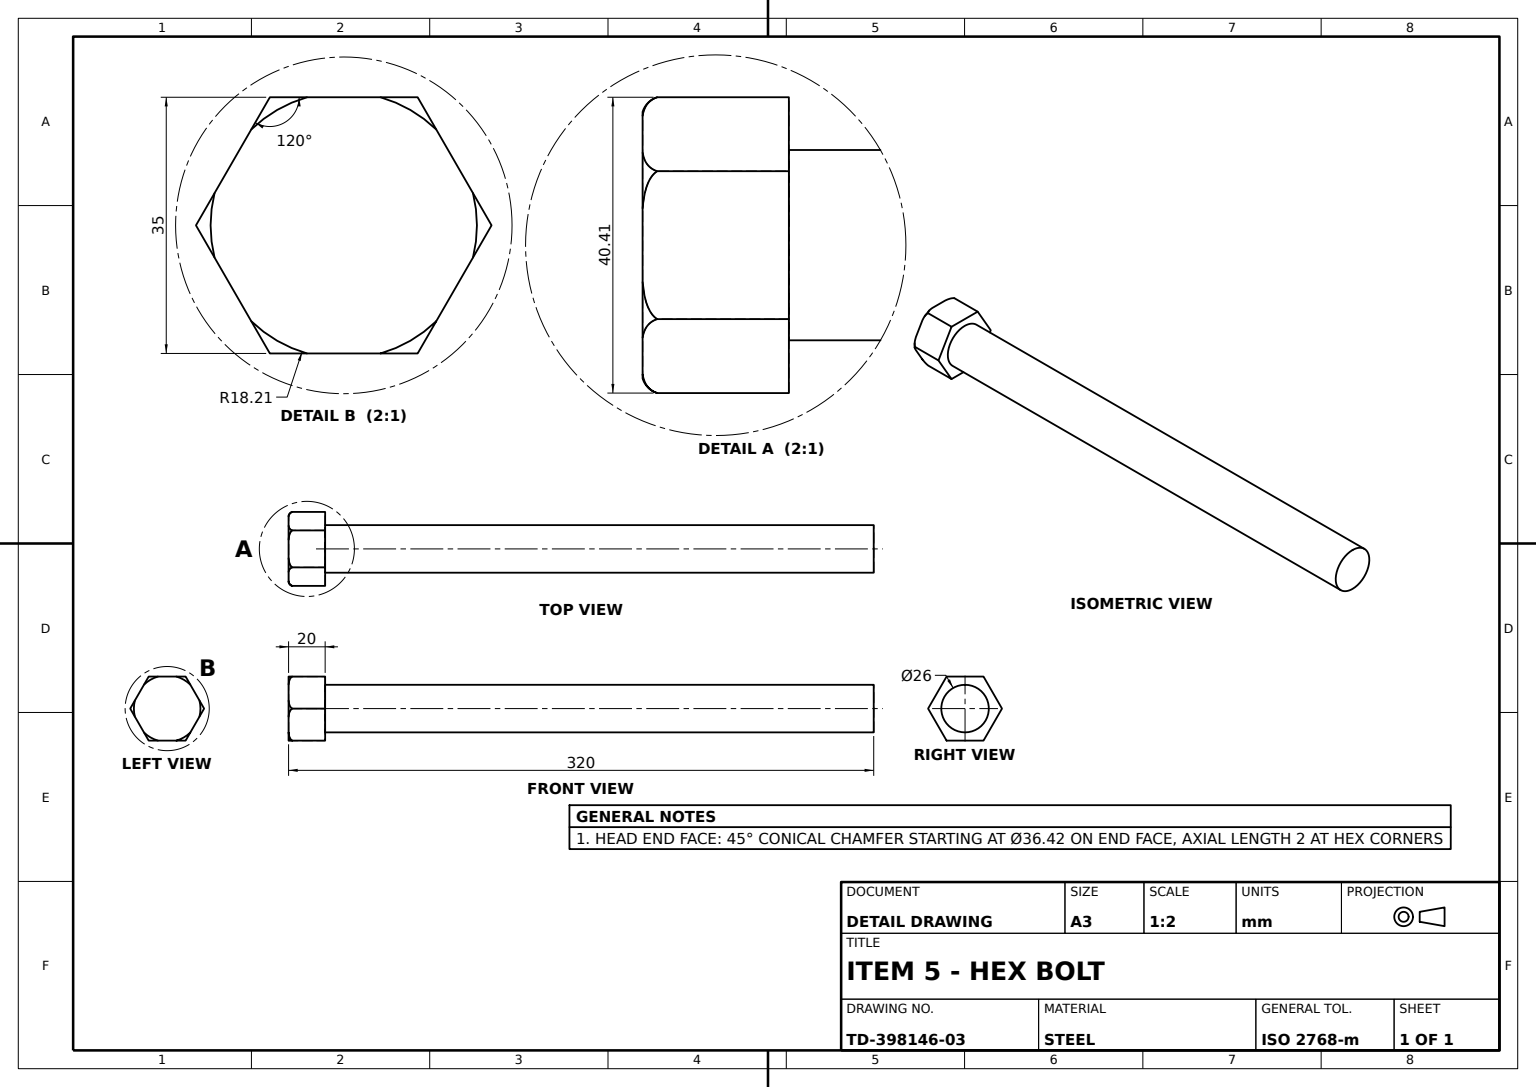
ISO-10303-21;
HEADER;
FILE_DESCRIPTION((''),'2;1');
FILE_NAME('','',(''),(''),'','','');
FILE_SCHEMA(('AUTOMOTIVE_DESIGN'));
ENDSEC;
DATA;
#1=APPLICATION_CONTEXT('');
#2=PRODUCT_CONTEXT('',#1,'mechanical');
#3=PRODUCT('','','',(#2));
#4=PRODUCT_DEFINITION_FORMATION('','',#3);
#5=PRODUCT_DEFINITION_CONTEXT('',#1,'design');
#6=PRODUCT_DEFINITION('','',#4,#5);
#7=PRODUCT_DEFINITION_SHAPE('','',#6);
#8=(LENGTH_UNIT()NAMED_UNIT(*)SI_UNIT(.MILLI.,.METRE.));
#9=(NAMED_UNIT(*)PLANE_ANGLE_UNIT()SI_UNIT($,.RADIAN.));
#10=(NAMED_UNIT(*)SI_UNIT($,.STERADIAN.)SOLID_ANGLE_UNIT());
#11=UNCERTAINTY_MEASURE_WITH_UNIT(LENGTH_MEASURE(1.E-05),#8,'distance_accuracy_value','');
#12=(GEOMETRIC_REPRESENTATION_CONTEXT(3)GLOBAL_UNCERTAINTY_ASSIGNED_CONTEXT((#11))GLOBAL_UNIT_ASSIGNED_CONTEXT((#8,#9,#10))REPRESENTATION_CONTEXT('',''));
#13=CARTESIAN_POINT('',(17.668127,20.,-4.397906));
#14=VERTEX_POINT('',#13);
#15=CARTESIAN_POINT('',(17.668127,20.,4.397906));
#16=VERTEX_POINT('',#15);
#17=CARTESIAN_POINT('',(0.,20.,0.));
#18=DIRECTION('',(0.,-1.,0.));
#19=DIRECTION('',(0.,0.,1.));
#20=AXIS2_PLACEMENT_3D('',#17,#18,#19);
#21=CIRCLE('',#20,18.207259);
#22=EDGE_CURVE('',#14,#16,#21,.T.);
#23=ORIENTED_EDGE('',*,*,#22,.T.);
#24=CARTESIAN_POINT('',(20.207259,18.,0.));
#25=VERTEX_POINT('',#24);
#26=CARTESIAN_POINT('',(20.145167,18.204696,0.107546));
#27=CARTESIAN_POINT('',(20.067875,18.380727,0.241421));
#28=CARTESIAN_POINT('',(19.893968,18.69635,0.542637));
#29=CARTESIAN_POINT('',(19.796459,18.835748,0.711527));
#30=CARTESIAN_POINT('',(19.594991,19.077372,1.06048));
#31=CARTESIAN_POINT('',(19.489991,19.181438,1.242345));
#32=CARTESIAN_POINT('',(19.273839,19.365421,1.616731));
#33=CARTESIAN_POINT('',(19.16218,19.445473,1.81013));
#34=CARTESIAN_POINT('',(18.825055,19.654439,2.394049));
#35=CARTESIAN_POINT('',(18.596554,19.754069,2.789824));
#36=CARTESIAN_POINT('',(18.135221,19.907509,3.588876));
#37=CARTESIAN_POINT('',(17.902338,19.960782,3.992241));
#38=B_SPLINE_CURVE_WITH_KNOTS('',3,(#24,#26,#27,#28,#29,#30,#31,#32,#33,#34,#35,#36,#37,#15),.UNSPECIFIED.,.F.,.F.,(4,2,2,2,2,2,4),(0.000000229,0.000702604,0.001404979,0.002107355,0.00280973,0.004214481,0.005619231),.UNSPECIFIED.);
#39=EDGE_CURVE('',#25,#16,#38,.T.);
#40=ORIENTED_EDGE('',*,*,#39,.F.);
#41=CARTESIAN_POINT('',(17.902082,19.960825,-3.992684));
#42=CARTESIAN_POINT('',(18.134693,19.907626,-3.58979));
#43=CARTESIAN_POINT('',(18.595438,19.754498,-2.791757));
#44=CARTESIAN_POINT('',(18.823622,19.655098,-2.396531));
#45=CARTESIAN_POINT('',(19.160225,19.446798,-1.813516));
#46=CARTESIAN_POINT('',(19.271845,19.366951,-1.620186));
#47=CARTESIAN_POINT('',(19.488371,19.182983,-1.245151));
#48=CARTESIAN_POINT('',(19.593676,19.078818,-1.062757));
#49=CARTESIAN_POINT('',(19.796013,18.836412,-0.7123));
#50=CARTESIAN_POINT('',(19.892647,18.698371,-0.544925));
#51=CARTESIAN_POINT('',(20.066575,18.383458,-0.243673));
#52=CARTESIAN_POINT('',(20.145542,18.203461,-0.106897));
#53=B_SPLINE_CURVE_WITH_KNOTS('',3,(#13,#41,#42,#43,#44,#45,#46,#47,#48,#49,#50,#51,#52,#24),.UNSPECIFIED.,.F.,.F.,(4,2,2,2,2,2,4),(0.000002385,0.001403147,0.002803908,0.003504289,0.004204669,0.00490505,0.005605431),.UNSPECIFIED.);
#54=EDGE_CURVE('',#14,#25,#53,.T.);
#55=ORIENTED_EDGE('',*,*,#54,.F.);
#56=EDGE_LOOP('',(#23,#40,#55));
#57=FACE_OUTER_BOUND('',#56,.T.);
#58=CARTESIAN_POINT('',(0.,17.129171,0.));
#59=DIRECTION('',(0.,0.,-1.));
#60=AXIS2_PLACEMENT_3D('',#58,#18,#59);
#61=TOROIDAL_SURFACE('',#60,17.336431,3.);
#62=ADVANCED_FACE('',(#57),#61,.T.);
#63=CARTESIAN_POINT('',(0.,0.,-13.));
#64=VERTEX_POINT('',#63);
#65=CARTESIAN_POINT('',(0.,0.,13.));
#66=VERTEX_POINT('',#65);
#67=CARTESIAN_POINT('',(0.,0.,0.));
#68=AXIS2_PLACEMENT_3D('',#67,#18,#59);
#69=CIRCLE('',#68,13.);
#70=EDGE_CURVE('',#64,#66,#69,.T.);
#71=ORIENTED_EDGE('',*,*,#70,.T.);
#72=CARTESIAN_POINT('',(0.,-300.,13.));
#73=VERTEX_POINT('',#72);
#74=DIRECTION('',(0.,1.,0.));
#75=VECTOR('',#74,1000.);
#76=LINE('',#72,#75);
#77=EDGE_CURVE('',#73,#66,#76,.T.);
#78=ORIENTED_EDGE('',*,*,#77,.F.);
#79=CARTESIAN_POINT('',(0.,-300.,-13.));
#80=VERTEX_POINT('',#79);
#81=CARTESIAN_POINT('',(0.,-300.,0.));
#82=AXIS2_PLACEMENT_3D('',#81,#18,#59);
#83=CIRCLE('',#82,13.);
#84=EDGE_CURVE('',#80,#73,#83,.T.);
#85=ORIENTED_EDGE('',*,*,#84,.F.);
#86=LINE('',#79,#75);
#87=EDGE_CURVE('',#80,#64,#86,.T.);
#88=ORIENTED_EDGE('',*,*,#87,.T.);
#89=EDGE_LOOP('',(#71,#78,#85,#88));
#90=FACE_OUTER_BOUND('',#89,.T.);
#91=AXIS2_PLACEMENT_3D('',#81,#74,#19);
#92=CYLINDRICAL_SURFACE('',#91,13.);
#93=ADVANCED_FACE('',(#90),#92,.T.);
#94=CARTESIAN_POINT('',(-5.025365,20.,17.5));
#95=VERTEX_POINT('',#94);
#96=CARTESIAN_POINT('',(-10.10363,18.,17.5));
#97=VERTEX_POINT('',#96);
#98=CARTESIAN_POINT('',(-5.492104,19.960923,17.5));
#99=CARTESIAN_POINT('',(-5.960143,19.907453,17.5));
#100=CARTESIAN_POINT('',(-6.884053,19.753721,17.5));
#101=CARTESIAN_POINT('',(-7.33942,19.654067,17.5));
#102=CARTESIAN_POINT('',(-8.006087,19.447914,17.5));
#103=CARTESIAN_POINT('',(-8.225551,19.369653,17.5));
#104=CARTESIAN_POINT('',(-8.65696,19.187123,17.5));
#105=CARTESIAN_POINT('',(-8.870751,19.081899,17.5));
#106=CARTESIAN_POINT('',(-9.277733,18.838784,17.5));
#107=CARTESIAN_POINT('',(-9.470105,18.701958,17.5));
#108=CARTESIAN_POINT('',(-9.822347,18.383681,17.5));
#109=CARTESIAN_POINT('',(-9.980357,18.203194,17.5));
#110=B_SPLINE_CURVE_WITH_KNOTS('',3,(#94,#98,#99,#100,#101,#102,#103,#104,#105,#106,#107,#108,#109,#96),.UNSPECIFIED.,.F.,.F.,(4,2,2,2,2,2,4),(0.00502645,0.006430133,0.007833817,0.008535659,0.009237501,0.009939343,0.010641184),.UNSPECIFIED.);
#111=EDGE_CURVE('',#95,#97,#110,.T.);
#112=ORIENTED_EDGE('',*,*,#111,.T.);
#113=CARTESIAN_POINT('',(-10.10363,0.,17.5));
#114=VERTEX_POINT('',#113);
#115=CARTESIAN_POINT('',(-10.10363,20.,17.5));
#116=VECTOR('',#18,1000.);
#117=LINE('',#115,#116);
#118=EDGE_CURVE('',#97,#114,#117,.T.);
#119=ORIENTED_EDGE('',*,*,#118,.T.);
#120=CARTESIAN_POINT('',(10.10363,0.,17.5));
#121=VERTEX_POINT('',#120);
#122=DIRECTION('',(1.,0.,0.));
#123=VECTOR('',#122,1000.);
#124=LINE('',#113,#123);
#125=EDGE_CURVE('',#114,#121,#124,.T.);
#126=ORIENTED_EDGE('',*,*,#125,.T.);
#127=CARTESIAN_POINT('',(10.10363,18.,17.5));
#128=VERTEX_POINT('',#127);
#129=CARTESIAN_POINT('',(10.10363,20.,17.5));
#130=LINE('',#129,#116);
#131=EDGE_CURVE('',#128,#121,#130,.T.);
#132=ORIENTED_EDGE('',*,*,#131,.F.);
#133=CARTESIAN_POINT('',(5.025365,20.,17.5));
#134=VERTEX_POINT('',#133);
#135=CARTESIAN_POINT('',(9.98061,18.202777,17.5));
#136=CARTESIAN_POINT('',(9.825141,18.380727,17.5));
#137=CARTESIAN_POINT('',(9.473221,18.699564,17.5));
#138=CARTESIAN_POINT('',(9.282037,18.835729,17.5));
#139=CARTESIAN_POINT('',(8.87945,19.077171,17.5));
#140=CARTESIAN_POINT('',(8.666501,19.182682,17.5));
#141=CARTESIAN_POINT('',(8.233223,19.366796,17.5));
#142=CARTESIAN_POINT('',(8.012779,19.445661,17.5));
#143=CARTESIAN_POINT('',(7.343094,19.653291,17.5));
#144=CARTESIAN_POINT('',(6.885612,19.753482,17.5));
#145=CARTESIAN_POINT('',(5.957388,19.90789,17.5));
#146=CARTESIAN_POINT('',(5.491532,19.960971,17.5));
#147=B_SPLINE_CURVE_WITH_KNOTS('',3,(#127,#135,#136,#137,#138,#139,#140,#141,#142,#143,#144,#145,#146,#133),.UNSPECIFIED.,.F.,.F.,(4,2,2,2,2,2,4),(0.035514707,0.036213744,0.036912782,0.037611819,0.038310856,0.039708931,0.041107005),.UNSPECIFIED.);
#148=EDGE_CURVE('',#128,#134,#147,.T.);
#149=ORIENTED_EDGE('',*,*,#148,.T.);
#150=LINE('',#115,#123);
#151=EDGE_CURVE('',#95,#134,#150,.T.);
#152=ORIENTED_EDGE('',*,*,#151,.F.);
#153=EDGE_LOOP('',(#112,#119,#126,#132,#149,#152));
#154=FACE_OUTER_BOUND('',#153,.T.);
#155=DIRECTION('',(-1.,0.,0.));
#156=AXIS2_PLACEMENT_3D('',#115,#59,#155);
#157=PLANE('',#156);
#158=ADVANCED_FACE('',(#154),#157,.F.);
#159=CARTESIAN_POINT('',(10.10363,18.,-17.5));
#160=VERTEX_POINT('',#159);
#161=CARTESIAN_POINT('',(10.10363,0.,-17.5));
#162=VERTEX_POINT('',#161);
#163=CARTESIAN_POINT('',(10.10363,20.,-17.5));
#164=LINE('',#163,#116);
#165=EDGE_CURVE('',#160,#162,#164,.T.);
#166=ORIENTED_EDGE('',*,*,#165,.F.);
#167=CARTESIAN_POINT('',(12.642762,20.,-13.102094));
#168=VERTEX_POINT('',#167);
#169=CARTESIAN_POINT('',(10.165722,18.204696,-17.392454));
#170=CARTESIAN_POINT('',(10.243014,18.380727,-17.258579));
#171=CARTESIAN_POINT('',(10.416921,18.69635,-16.957363));
#172=CARTESIAN_POINT('',(10.51443,18.835748,-16.788473));
#173=CARTESIAN_POINT('',(10.715898,19.077372,-16.43952));
#174=CARTESIAN_POINT('',(10.820898,19.181438,-16.257655));
#175=CARTESIAN_POINT('',(11.03705,19.365421,-15.883269));
#176=CARTESIAN_POINT('',(11.148709,19.445473,-15.68987));
#177=CARTESIAN_POINT('',(11.485835,19.654439,-15.105951));
#178=CARTESIAN_POINT('',(11.714336,19.754069,-14.710176));
#179=CARTESIAN_POINT('',(12.175668,19.907509,-13.911124));
#180=CARTESIAN_POINT('',(12.408551,19.960782,-13.507759));
#181=B_SPLINE_CURVE_WITH_KNOTS('',3,(#159,#169,#170,#171,#172,#173,#174,#175,#176,#177,#178,#179,#180,#167),.UNSPECIFIED.,.F.,.F.,(4,2,2,2,2,2,4),(0.000000229,0.000702604,0.001404979,0.002107355,0.00280973,0.004214481,0.005619231),.UNSPECIFIED.);
#182=EDGE_CURVE('',#160,#168,#181,.T.);
#183=ORIENTED_EDGE('',*,*,#182,.T.);
#184=CARTESIAN_POINT('',(20.207259,20.,0.));
#185=DIRECTION('',(-0.5,0.,-0.866025404));
#186=VECTOR('',#185,1000.);
#187=LINE('',#184,#186);
#188=EDGE_CURVE('',#14,#168,#187,.T.);
#189=ORIENTED_EDGE('',*,*,#188,.F.);
#190=ORIENTED_EDGE('',*,*,#54,.T.);
#191=CARTESIAN_POINT('',(20.207259,0.,0.));
#192=VERTEX_POINT('',#191);
#193=LINE('',#184,#116);
#194=EDGE_CURVE('',#25,#192,#193,.T.);
#195=ORIENTED_EDGE('',*,*,#194,.T.);
#196=LINE('',#191,#186);
#197=EDGE_CURVE('',#192,#162,#196,.T.);
#198=ORIENTED_EDGE('',*,*,#197,.T.);
#199=EDGE_LOOP('',(#166,#183,#189,#190,#195,#198));
#200=FACE_OUTER_BOUND('',#199,.T.);
#201=DIRECTION('',(-0.866025404,0.,0.5));
#202=DIRECTION('',(0.5,0.,0.866025404));
#203=AXIS2_PLACEMENT_3D('',#184,#201,#202);
#204=PLANE('',#203);
#205=ADVANCED_FACE('',(#200),#204,.F.);
#206=CARTESIAN_POINT('',(-20.207259,18.,0.));
#207=VERTEX_POINT('',#206);
#208=CARTESIAN_POINT('',(-20.207259,0.,0.));
#209=VERTEX_POINT('',#208);
#210=CARTESIAN_POINT('',(-20.207259,20.,0.));
#211=LINE('',#210,#116);
#212=EDGE_CURVE('',#207,#209,#211,.T.);
#213=ORIENTED_EDGE('',*,*,#212,.F.);
#214=CARTESIAN_POINT('',(-17.668127,20.,-4.397906));
#215=VERTEX_POINT('',#214);
#216=CARTESIAN_POINT('',(-20.145167,18.204696,-0.107546));
#217=CARTESIAN_POINT('',(-20.067875,18.380727,-0.241421));
#218=CARTESIAN_POINT('',(-19.893968,18.69635,-0.542637));
#219=CARTESIAN_POINT('',(-19.796459,18.835748,-0.711527));
#220=CARTESIAN_POINT('',(-19.594991,19.077372,-1.06048));
#221=CARTESIAN_POINT('',(-19.489991,19.181438,-1.242345));
#222=CARTESIAN_POINT('',(-19.273839,19.365421,-1.616731));
#223=CARTESIAN_POINT('',(-19.16218,19.445473,-1.81013));
#224=CARTESIAN_POINT('',(-18.825055,19.654439,-2.394049));
#225=CARTESIAN_POINT('',(-18.596554,19.754069,-2.789824));
#226=CARTESIAN_POINT('',(-18.135221,19.907509,-3.588876));
#227=CARTESIAN_POINT('',(-17.902338,19.960782,-3.992241));
#228=B_SPLINE_CURVE_WITH_KNOTS('',3,(#206,#216,#217,#218,#219,#220,#221,#222,#223,#224,#225,#226,#227,#214),.UNSPECIFIED.,.F.,.F.,(4,2,2,2,2,2,4),(0.000000229,0.000702604,0.001404979,0.002107355,0.00280973,0.004214481,0.005619231),.UNSPECIFIED.);
#229=EDGE_CURVE('',#207,#215,#228,.T.);
#230=ORIENTED_EDGE('',*,*,#229,.T.);
#231=CARTESIAN_POINT('',(-12.642762,20.,-13.102094));
#232=VERTEX_POINT('',#231);
#233=CARTESIAN_POINT('',(-10.10363,20.,-17.5));
#234=DIRECTION('',(-0.5,0.,0.866025404));
#235=VECTOR('',#234,1000.);
#236=LINE('',#233,#235);
#237=EDGE_CURVE('',#232,#215,#236,.T.);
#238=ORIENTED_EDGE('',*,*,#237,.F.);
#239=CARTESIAN_POINT('',(-10.10363,18.,-17.5));
#240=VERTEX_POINT('',#239);
#241=CARTESIAN_POINT('',(-12.408807,19.960825,-13.507316));
#242=CARTESIAN_POINT('',(-12.176196,19.907626,-13.91021));
#243=CARTESIAN_POINT('',(-11.715451,19.754498,-14.708243));
#244=CARTESIAN_POINT('',(-11.487267,19.655098,-15.103469));
#245=CARTESIAN_POINT('',(-11.150664,19.446798,-15.686484));
#246=CARTESIAN_POINT('',(-11.039045,19.366951,-15.879814));
#247=CARTESIAN_POINT('',(-10.822518,19.182983,-16.254849));
#248=CARTESIAN_POINT('',(-10.717213,19.078818,-16.437243));
#249=CARTESIAN_POINT('',(-10.514876,18.836412,-16.7877));
#250=CARTESIAN_POINT('',(-10.418243,18.698371,-16.955075));
#251=CARTESIAN_POINT('',(-10.244314,18.383458,-17.256327));
#252=CARTESIAN_POINT('',(-10.165347,18.203461,-17.393103));
#253=B_SPLINE_CURVE_WITH_KNOTS('',3,(#231,#241,#242,#243,#244,#245,#246,#247,#248,#249,#250,#251,#252,#239),.UNSPECIFIED.,.F.,.F.,(4,2,2,2,2,2,4),(0.000002385,0.001403147,0.002803908,0.003504289,0.004204669,0.00490505,0.005605431),.UNSPECIFIED.);
#254=EDGE_CURVE('',#232,#240,#253,.T.);
#255=ORIENTED_EDGE('',*,*,#254,.T.);
#256=CARTESIAN_POINT('',(-10.10363,0.,-17.5));
#257=VERTEX_POINT('',#256);
#258=LINE('',#233,#116);
#259=EDGE_CURVE('',#240,#257,#258,.T.);
#260=ORIENTED_EDGE('',*,*,#259,.T.);
#261=LINE('',#256,#235);
#262=EDGE_CURVE('',#257,#209,#261,.T.);
#263=ORIENTED_EDGE('',*,*,#262,.T.);
#264=EDGE_LOOP('',(#213,#230,#238,#255,#260,#263));
#265=FACE_OUTER_BOUND('',#264,.T.);
#266=DIRECTION('',(0.866025404,0.,0.5));
#267=DIRECTION('',(0.5,0.,-0.866025404));
#268=AXIS2_PLACEMENT_3D('',#233,#266,#267);
#269=PLANE('',#268);
#270=ADVANCED_FACE('',(#265),#269,.F.);
#271=ORIENTED_EDGE('',*,*,#39,.T.);
#272=CARTESIAN_POINT('',(12.642762,20.,13.102094));
#273=VERTEX_POINT('',#272);
#274=VECTOR('',#267,1000.);
#275=LINE('',#129,#274);
#276=EDGE_CURVE('',#273,#16,#275,.T.);
#277=ORIENTED_EDGE('',*,*,#276,.F.);
#278=CARTESIAN_POINT('',(12.408807,19.960825,13.507316));
#279=CARTESIAN_POINT('',(12.176196,19.907626,13.91021));
#280=CARTESIAN_POINT('',(11.715451,19.754498,14.708243));
#281=CARTESIAN_POINT('',(11.487267,19.655098,15.103469));
#282=CARTESIAN_POINT('',(11.150664,19.446798,15.686484));
#283=CARTESIAN_POINT('',(11.039045,19.366951,15.879814));
#284=CARTESIAN_POINT('',(10.822518,19.182983,16.254849));
#285=CARTESIAN_POINT('',(10.717213,19.078818,16.437243));
#286=CARTESIAN_POINT('',(10.514876,18.836412,16.7877));
#287=CARTESIAN_POINT('',(10.418243,18.698371,16.955075));
#288=CARTESIAN_POINT('',(10.244314,18.383458,17.256327));
#289=CARTESIAN_POINT('',(10.165347,18.203461,17.393103));
#290=B_SPLINE_CURVE_WITH_KNOTS('',3,(#272,#278,#279,#280,#281,#282,#283,#284,#285,#286,#287,#288,#289,#127),.UNSPECIFIED.,.F.,.F.,(4,2,2,2,2,2,4),(0.000002385,0.001403147,0.002803908,0.003504289,0.004204669,0.00490505,0.005605431),.UNSPECIFIED.);
#291=EDGE_CURVE('',#273,#128,#290,.T.);
#292=ORIENTED_EDGE('',*,*,#291,.T.);
#293=ORIENTED_EDGE('',*,*,#131,.T.);
#294=LINE('',#120,#274);
#295=EDGE_CURVE('',#121,#192,#294,.T.);
#296=ORIENTED_EDGE('',*,*,#295,.T.);
#297=ORIENTED_EDGE('',*,*,#194,.F.);
#298=EDGE_LOOP('',(#271,#277,#292,#293,#296,#297));
#299=FACE_OUTER_BOUND('',#298,.T.);
#300=DIRECTION('',(-0.866025404,0.,-0.5));
#301=AXIS2_PLACEMENT_3D('',#129,#300,#234);
#302=PLANE('',#301);
#303=ADVANCED_FACE('',(#299),#302,.F.);
#304=EDGE_CURVE('',#73,#80,#83,.T.);
#305=ORIENTED_EDGE('',*,*,#304,.F.);
#306=ORIENTED_EDGE('',*,*,#77,.T.);
#307=EDGE_CURVE('',#66,#64,#69,.T.);
#308=ORIENTED_EDGE('',*,*,#307,.T.);
#309=ORIENTED_EDGE('',*,*,#87,.F.);
#310=EDGE_LOOP('',(#305,#306,#308,#309));
#311=FACE_OUTER_BOUND('',#310,.T.);
#312=ADVANCED_FACE('',(#311),#92,.T.);
#313=CARTESIAN_POINT('',(-12.642762,20.,13.102094));
#314=VERTEX_POINT('',#313);
#315=EDGE_CURVE('',#95,#314,#21,.T.);
#316=ORIENTED_EDGE('',*,*,#315,.T.);
#317=CARTESIAN_POINT('',(-10.165722,18.204696,17.392454));
#318=CARTESIAN_POINT('',(-10.243014,18.380727,17.258579));
#319=CARTESIAN_POINT('',(-10.416921,18.69635,16.957363));
#320=CARTESIAN_POINT('',(-10.51443,18.835748,16.788473));
#321=CARTESIAN_POINT('',(-10.715898,19.077372,16.43952));
#322=CARTESIAN_POINT('',(-10.820898,19.181438,16.257655));
#323=CARTESIAN_POINT('',(-11.03705,19.365421,15.883269));
#324=CARTESIAN_POINT('',(-11.148709,19.445473,15.68987));
#325=CARTESIAN_POINT('',(-11.485835,19.654439,15.105951));
#326=CARTESIAN_POINT('',(-11.714336,19.754069,14.710176));
#327=CARTESIAN_POINT('',(-12.175668,19.907509,13.911124));
#328=CARTESIAN_POINT('',(-12.408551,19.960782,13.507759));
#329=B_SPLINE_CURVE_WITH_KNOTS('',3,(#96,#317,#318,#319,#320,#321,#322,#323,#324,#325,#326,#327,#328,#313),.UNSPECIFIED.,.F.,.F.,(4,2,2,2,2,2,4),(0.000000229,0.000702604,0.001404979,0.002107355,0.00280973,0.004214481,0.005619231),.UNSPECIFIED.);
#330=EDGE_CURVE('',#97,#314,#329,.T.);
#331=ORIENTED_EDGE('',*,*,#330,.F.);
#332=ORIENTED_EDGE('',*,*,#111,.F.);
#333=EDGE_LOOP('',(#316,#331,#332));
#334=FACE_OUTER_BOUND('',#333,.T.);
#335=ADVANCED_FACE('',(#334),#61,.T.);
#336=VECTOR('',#202,1000.);
#337=LINE('',#208,#336);
#338=EDGE_CURVE('',#209,#114,#337,.T.);
#339=ORIENTED_EDGE('',*,*,#338,.T.);
#340=ORIENTED_EDGE('',*,*,#118,.F.);
#341=ORIENTED_EDGE('',*,*,#330,.T.);
#342=CARTESIAN_POINT('',(-17.668127,20.,4.397906));
#343=VERTEX_POINT('',#342);
#344=LINE('',#210,#336);
#345=EDGE_CURVE('',#343,#314,#344,.T.);
#346=ORIENTED_EDGE('',*,*,#345,.F.);
#347=CARTESIAN_POINT('',(-17.902082,19.960825,3.992684));
#348=CARTESIAN_POINT('',(-18.134693,19.907626,3.58979));
#349=CARTESIAN_POINT('',(-18.595438,19.754498,2.791757));
#350=CARTESIAN_POINT('',(-18.823622,19.655098,2.396531));
#351=CARTESIAN_POINT('',(-19.160225,19.446798,1.813516));
#352=CARTESIAN_POINT('',(-19.271845,19.366951,1.620186));
#353=CARTESIAN_POINT('',(-19.488371,19.182983,1.245151));
#354=CARTESIAN_POINT('',(-19.593676,19.078818,1.062757));
#355=CARTESIAN_POINT('',(-19.796013,18.836412,0.7123));
#356=CARTESIAN_POINT('',(-19.892647,18.698371,0.544925));
#357=CARTESIAN_POINT('',(-20.066575,18.383458,0.243673));
#358=CARTESIAN_POINT('',(-20.145542,18.203461,0.106897));
#359=B_SPLINE_CURVE_WITH_KNOTS('',3,(#342,#347,#348,#349,#350,#351,#352,#353,#354,#355,#356,#357,#358,#206),.UNSPECIFIED.,.F.,.F.,(4,2,2,2,2,2,4),(0.000002385,0.001403147,0.002803908,0.003504289,0.004204669,0.00490505,0.005605431),.UNSPECIFIED.);
#360=EDGE_CURVE('',#343,#207,#359,.T.);
#361=ORIENTED_EDGE('',*,*,#360,.T.);
#362=ORIENTED_EDGE('',*,*,#212,.T.);
#363=EDGE_LOOP('',(#339,#340,#341,#346,#361,#362));
#364=FACE_OUTER_BOUND('',#363,.T.);
#365=DIRECTION('',(0.866025404,0.,-0.5));
#366=AXIS2_PLACEMENT_3D('',#210,#365,#185);
#367=PLANE('',#366);
#368=ADVANCED_FACE('',(#364),#367,.F.);
#369=ORIENTED_EDGE('',*,*,#254,.F.);
#370=CARTESIAN_POINT('',(-5.025365,20.,-17.5));
#371=VERTEX_POINT('',#370);
#372=EDGE_CURVE('',#232,#371,#21,.T.);
#373=ORIENTED_EDGE('',*,*,#372,.T.);
#374=CARTESIAN_POINT('',(-9.98061,18.202777,-17.5));
#375=CARTESIAN_POINT('',(-9.825141,18.380727,-17.5));
#376=CARTESIAN_POINT('',(-9.473221,18.699564,-17.5));
#377=CARTESIAN_POINT('',(-9.282037,18.835729,-17.5));
#378=CARTESIAN_POINT('',(-8.87945,19.077171,-17.5));
#379=CARTESIAN_POINT('',(-8.666501,19.182682,-17.5));
#380=CARTESIAN_POINT('',(-8.233223,19.366796,-17.5));
#381=CARTESIAN_POINT('',(-8.012779,19.445661,-17.5));
#382=CARTESIAN_POINT('',(-7.343094,19.653291,-17.5));
#383=CARTESIAN_POINT('',(-6.885612,19.753482,-17.5));
#384=CARTESIAN_POINT('',(-5.957388,19.90789,-17.5));
#385=CARTESIAN_POINT('',(-5.491532,19.960971,-17.5));
#386=B_SPLINE_CURVE_WITH_KNOTS('',3,(#239,#374,#375,#376,#377,#378,#379,#380,#381,#382,#383,#384,#385,#370),.UNSPECIFIED.,.F.,.F.,(4,2,2,2,2,2,4),(0.035514707,0.036213744,0.036912782,0.037611819,0.038310856,0.039708931,0.041107005),.UNSPECIFIED.);
#387=EDGE_CURVE('',#240,#371,#386,.T.);
#388=ORIENTED_EDGE('',*,*,#387,.F.);
#389=EDGE_LOOP('',(#369,#373,#388));
#390=FACE_OUTER_BOUND('',#389,.T.);
#391=ADVANCED_FACE('',(#390),#61,.T.);
#392=ORIENTED_EDGE('',*,*,#70,.F.);
#393=ORIENTED_EDGE('',*,*,#307,.F.);
#394=EDGE_LOOP('',(#392,#393));
#395=FACE_BOUND('',#394,.T.);
#396=ORIENTED_EDGE('',*,*,#338,.F.);
#397=ORIENTED_EDGE('',*,*,#262,.F.);
#398=VECTOR('',#155,1000.);
#399=LINE('',#161,#398);
#400=EDGE_CURVE('',#162,#257,#399,.T.);
#401=ORIENTED_EDGE('',*,*,#400,.F.);
#402=ORIENTED_EDGE('',*,*,#197,.F.);
#403=ORIENTED_EDGE('',*,*,#295,.F.);
#404=ORIENTED_EDGE('',*,*,#125,.F.);
#405=EDGE_LOOP('',(#396,#397,#401,#402,#403,#404));
#406=FACE_OUTER_BOUND('',#405,.T.);
#407=AXIS2_PLACEMENT_3D('',#67,#74,#19);
#408=PLANE('',#407);
#409=ADVANCED_FACE('',(#395,#406),#408,.F.);
#410=ORIENTED_EDGE('',*,*,#259,.F.);
#411=ORIENTED_EDGE('',*,*,#387,.T.);
#412=CARTESIAN_POINT('',(5.025365,20.,-17.5));
#413=VERTEX_POINT('',#412);
#414=LINE('',#163,#398);
#415=EDGE_CURVE('',#413,#371,#414,.T.);
#416=ORIENTED_EDGE('',*,*,#415,.F.);
#417=CARTESIAN_POINT('',(5.492104,19.960923,-17.5));
#418=CARTESIAN_POINT('',(5.960143,19.907453,-17.5));
#419=CARTESIAN_POINT('',(6.884053,19.753721,-17.5));
#420=CARTESIAN_POINT('',(7.33942,19.654067,-17.5));
#421=CARTESIAN_POINT('',(8.006087,19.447914,-17.5));
#422=CARTESIAN_POINT('',(8.225551,19.369653,-17.5));
#423=CARTESIAN_POINT('',(8.65696,19.187123,-17.5));
#424=CARTESIAN_POINT('',(8.870751,19.081899,-17.5));
#425=CARTESIAN_POINT('',(9.277733,18.838784,-17.5));
#426=CARTESIAN_POINT('',(9.470105,18.701958,-17.5));
#427=CARTESIAN_POINT('',(9.822347,18.383681,-17.5));
#428=CARTESIAN_POINT('',(9.980357,18.203194,-17.5));
#429=B_SPLINE_CURVE_WITH_KNOTS('',3,(#412,#417,#418,#419,#420,#421,#422,#423,#424,#425,#426,#427,#428,#159),.UNSPECIFIED.,.F.,.F.,(4,2,2,2,2,2,4),(0.00502645,0.006430133,0.007833817,0.008535659,0.009237501,0.009939343,0.010641184),.UNSPECIFIED.);
#430=EDGE_CURVE('',#413,#160,#429,.T.);
#431=ORIENTED_EDGE('',*,*,#430,.T.);
#432=ORIENTED_EDGE('',*,*,#165,.T.);
#433=ORIENTED_EDGE('',*,*,#400,.T.);
#434=EDGE_LOOP('',(#410,#411,#416,#431,#432,#433));
#435=FACE_OUTER_BOUND('',#434,.T.);
#436=AXIS2_PLACEMENT_3D('',#163,#19,#122);
#437=PLANE('',#436);
#438=ADVANCED_FACE('',(#435),#437,.F.);
#439=EDGE_CURVE('',#273,#134,#21,.T.);
#440=ORIENTED_EDGE('',*,*,#439,.F.);
#441=ORIENTED_EDGE('',*,*,#276,.T.);
#442=ORIENTED_EDGE('',*,*,#22,.F.);
#443=ORIENTED_EDGE('',*,*,#188,.T.);
#444=AXIS2_PLACEMENT_3D('',#17,#18,#59);
#445=CIRCLE('',#444,18.207259);
#446=EDGE_CURVE('',#413,#168,#445,.T.);
#447=ORIENTED_EDGE('',*,*,#446,.F.);
#448=ORIENTED_EDGE('',*,*,#415,.T.);
#449=ORIENTED_EDGE('',*,*,#372,.F.);
#450=ORIENTED_EDGE('',*,*,#237,.T.);
#451=EDGE_CURVE('',#343,#215,#21,.T.);
#452=ORIENTED_EDGE('',*,*,#451,.F.);
#453=ORIENTED_EDGE('',*,*,#345,.T.);
#454=ORIENTED_EDGE('',*,*,#315,.F.);
#455=ORIENTED_EDGE('',*,*,#151,.T.);
#456=EDGE_LOOP('',(#440,#441,#442,#443,#447,#448,#449,#450,#452,#453,#454,#455));
#457=FACE_OUTER_BOUND('',#456,.T.);
#458=AXIS2_PLACEMENT_3D('',#17,#74,#19);
#459=PLANE('',#458);
#460=ADVANCED_FACE('',(#457),#459,.T.);
#461=ORIENTED_EDGE('',*,*,#229,.F.);
#462=ORIENTED_EDGE('',*,*,#360,.F.);
#463=ORIENTED_EDGE('',*,*,#451,.T.);
#464=EDGE_LOOP('',(#461,#462,#463));
#465=FACE_OUTER_BOUND('',#464,.T.);
#466=ADVANCED_FACE('',(#465),#61,.T.);
#467=ORIENTED_EDGE('',*,*,#430,.F.);
#468=ORIENTED_EDGE('',*,*,#446,.T.);
#469=ORIENTED_EDGE('',*,*,#182,.F.);
#470=EDGE_LOOP('',(#467,#468,#469));
#471=FACE_OUTER_BOUND('',#470,.T.);
#472=ADVANCED_FACE('',(#471),#61,.T.);
#473=ORIENTED_EDGE('',*,*,#304,.T.);
#474=ORIENTED_EDGE('',*,*,#84,.T.);
#475=EDGE_LOOP('',(#473,#474));
#476=FACE_OUTER_BOUND('',#475,.T.);
#477=PLANE('',#82);
#478=ADVANCED_FACE('',(#476),#477,.T.);
#479=ORIENTED_EDGE('',*,*,#291,.F.);
#480=ORIENTED_EDGE('',*,*,#439,.T.);
#481=ORIENTED_EDGE('',*,*,#148,.F.);
#482=EDGE_LOOP('',(#479,#480,#481));
#483=FACE_OUTER_BOUND('',#482,.T.);
#484=ADVANCED_FACE('',(#483),#61,.T.);
#485=CLOSED_SHELL('',(#62,#93,#158,#205,#270,#303,#312,#335,#368,#391,#409,#438,#460,#466,#472,#478,#484));
#486=MANIFOLD_SOLID_BREP('',#485);
#487=ADVANCED_BREP_SHAPE_REPRESENTATION('',(#486),#12);
#488=SHAPE_DEFINITION_REPRESENTATION(#7,#487);
ENDSEC;
END-ISO-10303-21;
